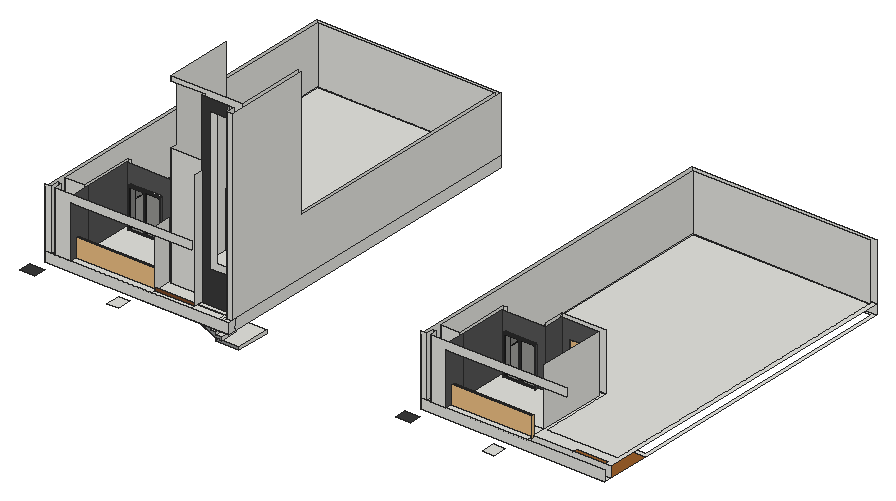
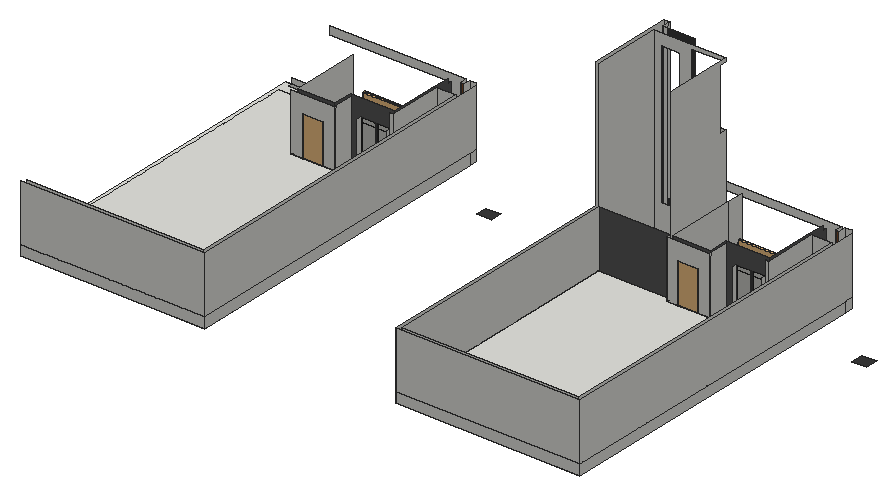
# SketchUp Ruby script. Lengths in inches.
U = 1.inch
M = Sketchup.active_model
def pt(a) = Geom::Point3d.new(a.map { |v| v * U })
def face(e, loops, mat)
  f = e.add_face(loops[0].map { |a| pt(a) })
  loops[1..].each { |l| e.add_face(l.map { |a| pt(a) }).erase! }
  f.material = f.back_material = mat if mat
  f
end
# faces: each face lists its corners as indices into pts; further lists are holes
def faces(e, pts, list, mat = nil) = list.each { |f| face(e, (f[0].is_a?(Array) ? f : [f]).map { |l| l.map { |i| pts[i] } }, mat) }
# xy, xz, yz: faces in a plane at the given z, y or x. An outline is a flat list of corners, or four numbers for a rectangle; further outlines are holes
def ring(l) = l.size == 4 ? [[l[0], l[1]], [l[2], l[1]], [l[2], l[3]], [l[0], l[3]]] : l.each_slice(2).to_a
def flat(e, list, mat, &to3) = list.each { |f| face(e, (f[0].is_a?(Array) ? f : [f]).map { |l| ring(l).map { |u, v| to3.(u, v) } }, mat) }
def xy(e, z, list, mat = nil) = flat(e, list, mat) { |x, y| [x, y, z] }
def xz(e, y, list, mat = nil) = flat(e, list, mat) { |x, z| [x, y, z] }
def yz(e, x, list, mat = nil) = flat(e, list, mat) { |y, z| [x, y, z] }
def lines(e, pts, list) = list.each { |a, b| e.add_line(pt(pts[a]), pt(pts[b])) }
# prism: a flat outline (further loops are holes) pulled along v
def prism(e, loops, v, mat = nil)
  f = face(e, loops, mat); d = Geom::Vector3d.new(v.map { |x| x * U })
  f.pushpull(f.normal.samedirection?(d) ? d.length : -d.length)
end
def box(e, o, s, mat = nil) = prism(e, [[o, [o[0] + s[0], o[1], o[2]], [o[0] + s[0], o[1] + s[1], o[2]], [o[0], o[1] + s[1], o[2]]]], [0, 0, s[2]], mat)
def at(x, y, z, deg = 0) = Geom::Transformation.translation(pt([x, y, z])) * Geom::Transformation.rotation(ORIGIN, Z_AXIS, deg.degrees)
def axes(o, x, y, z) = Geom::Transformation.new([*x, 0, *y, 0, *z, 0, *pt(o).to_a, 1])
def part(name) = M.definitions.add(name)
# library, detail: a bought-in or finely detailed component or shape, given as its bounding box
def library(name, o, s) = part(name).tap { |d| box(d.entities, o, s) }
def detail(e, o, s) = box(e.add_group.entities, o, s)
def put(e, d, t, mat = nil) = e.add_instance(d, t).tap { |i| i.material = mat if mat }
def group(e, t, mat = nil) = e.add_group.tap { |g| g.transformation = t; g.material = mat if mat }.entities
root = M.entities
M.materials.add("Glass_Tinted_Gray").color = [0, 0, 0]
M.materials["Glass_Tinted_Gray"].alpha = 0.125
M.materials.add("[0135_DarkGray]").color = [81, 81, 81]
M.materials.add("[Blacktop Old 02]").color = [143, 145, 145]
M.materials.add("[Color M06]").color = [86, 86, 86]
M.materials.add("[Color M07]").color = [58, 58, 58]
M.materials.add("[Mirror 02]").color = [229, 229, 229]
M.materials.add("[Terrazzo Light Blue]").color = [196, 214, 227]
M.materials.add("[Wood Floor Dark]").color = [153, 94, 42]
M.materials.add("[Wood Veneer 01]").color = [120, 70, 37]
c1 = part("PENTEK_RP Fineline 50S_Sliding_DoorCase_E1")
box(c1.entities,[0,0,0],[1.51,3.66,99.27],"[0135_DarkGray]")
c2 = part("PENTEK_RP Fineline 50S_SlidingDooe_Case_E2")
box(c2.entities,[0,0,0],[96.25,3.66,1.51],"[0135_DarkGray]")
c3 = part("pentek_RP Fineline 50S_SlidingDoor_Case")
put(c3.entities,c1,at(97.76,0,0))
put(c3.entities,c2,at(1.51,0,0))
put(c3.entities,c1,at(0,0,0))
put(c3.entities,c2,at(1.51,0,97.76))
c4 = part("PENTEK_RP Fineline 50S_SlidingDoor_GlazingBead_2")
box(c4.entities,[0,0,0],[0.56,0.59,94.39],"[0135_DarkGray]")
c5 = part("PENTEK_RP Fineline 50S_SlidingDoor_Glass")
box(c5.entities,[0,0,0],[46.58,0.16,94.39],"Glass_Tinted_Gray")
c6 = part("PENTEK_RP Fineline 50S_SlidingDoor_GlazingBead")
box(c6.entities,[0,0,0],[45.47,0.59,0.56],"[0135_DarkGray]")
c7 = part("PENTEK_RP Fineline 50S_SlidingDoor_Leaf_E1")
xy(c7.entities,0,[[0,0,0.93,1.97],[0.93,1.57,1.49,1.97]],"[0135_DarkGray]")
xy(c7.entities,96.25,[[0,0,0.93,0,0.93,1.57,1.49,1.57,1.49,1.97,0,1.97]],"[0135_DarkGray]")
xz(c7.entities,0,[[0,0,0.93,96.25]],"[0135_DarkGray]")
xz(c7.entities,1.57,[[0.93,0,1.49,95.32],[0.93,95.32,1.49,96.25]],"[0135_DarkGray]")
xz(c7.entities,1.97,[[0,0,1.49,96.25]],"[0135_DarkGray]")
yz(c7.entities,0,[[0,0,1.97,96.25]],"[0135_DarkGray]")
yz(c7.entities,0.93,[[0,0,1.57,0.93],[0,0.93,1.57,95.32],[0,95.32,1.57,96.25]],"[0135_DarkGray]")
yz(c7.entities,1.49,[[1.57,0,1.97,95.32],[1.57,95.32,1.97,96.25]],"[0135_DarkGray]")
c8 = part("PENTEK_RP Fineline 50S_SlidingDoor_Leaf_E2")
xy(c8.entities,0,[[0,0,0,1.57,0.56,1.57,0.56,1.97,46.02,1.97,46.02,1.57,46.58,1.57,46.58,0]],"[0135_DarkGray]")
xy(c8.entities,0.93,[[0,0,46.58,1.57]],"[0135_DarkGray]")
xy(c8.entities,1.49,[[0.56,1.57,46.02,1.97]],"[0135_DarkGray]")
xz(c8.entities,0,[[0,0,46.58,0.93]],"[0135_DarkGray]")
xz(c8.entities,1.57,[[0,0,0.56,0.93],[46.02,0,46.58,0.93],[0.56,0.93,46.02,1.49]],"[0135_DarkGray]")
xz(c8.entities,1.97,[[0.56,0,46.02,1.49]],"[0135_DarkGray]")
yz(c8.entities,0,[[0,0,1.57,0.93]],"[0135_DarkGray]")
yz(c8.entities,0.56,[[1.57,0,1.97,0.93],[1.57,0.93,1.97,1.49]],"[0135_DarkGray]")
yz(c8.entities,46.02,[[1.57,0,1.97,0.93],[1.57,0.93,1.97,1.49]],"[0135_DarkGray]")
yz(c8.entities,46.58,[[0,0,1.57,0.93]],"[0135_DarkGray]")
c9 = part("PENTEK_RP Fineline S_SlidingDoor_Leaf1")
put(c9.entities,c4,at(0.93,0,0.93))
put(c9.entities,c4,at(46.96,0,0.93))
put(c9.entities,c5,at(1.49,1.42,0.93))
put(c9.entities,c6,at(1.49,0,0.93))
put(c9.entities,c5,at(1.49,0.59,0.93),"[Terrazzo Light Blue]")
put(c9.entities,c7,at(0,0,0))
put(c9.entities,c7,axes([48.44,0,0],[-1,0,0],[0,1,0],[0,0,1]))
put(c9.entities,c8,axes([0.93,0,96.25],[1,0,0],[0,1,0],[0,0,-1]))
put(c9.entities,c8,at(0.93,0,0))
put(c9.entities,c6,at(1.49,0,94.77))
c10 = part("PENTEK_RP Fineline 50S_SlidingDoor_Leaf2")
put(c10.entities,c5,at(1.49,1.42,0.93))
put(c10.entities,c6,at(1.49,0,94.77))
put(c10.entities,c4,at(46.96,0,0.93))
put(c10.entities,c5,at(1.49,0.59,0.93),"[Mirror 02]")
put(c10.entities,c4,at(0.93,0,0.93))
put(c10.entities,c7,at(0,0,0))
put(c10.entities,c7,axes([48.44,0,0],[-1,0,0],[0,1,0],[0,0,1]))
put(c10.entities,c6,at(1.49,0,0.93))
put(c10.entities,c8,axes([0.93,0,96.25],[1,0,0],[0,1,0],[0,0,-1]))
put(c10.entities,c8,at(0.93,0,0))
c11 = part("PENTEK - Slimmest Steel Sliding Door / Window\#1")
put(c11.entities,c3,at(0,-1.88,-0.09))
put(c11.entities,c9,at(1.51,-2.27,1.42))
put(c11.entities,c10,at(49.32,-0.3,1.42))
c12 = library("Glass Railing",[0,0,0],[139.5,4.76,42])
c13 = library("door (1)",[38.93,25.48,0],[40,9.94,82.68])
xy(root,69.625,[[978.32,297.1875,1002.07,327.09],[1764.69,297.1875,1788.44,327.09]])
xy(root,69.625,[[796.71,297,827.45,321.97],[1583.09,297,1613.83,321.97]],"[Color M07]")
xy(root,71.875,[[1181.03,335.33,1193.03,371.33]])
xy(root,77.875,[[1205.03,299.33,1205.03,335.33,1217.03,335.33,1217.03,371.33,1253.03,371.33,1253.03,299.33],[1193.03,335.33,1205.03,371.33]])
xy(root,83.875,[[1205.03,299.33,1217.03,335.33],[1217.03,299.33,1253.03,299.33,1253.03,371.33,1205.03,371.33,1205.03,335.33,1217.03,335.33]])
xy(root,89.875,[[1205.03,299.33,1217.03,335.33]])
xy(root,94.0625,[[922.05,431.33,983.8,440.27],[1708.43,431.33,1770.18,440.27]])
xy(root,95.875,[[1193.03,299.33,1205.03,335.33]])
xy(root,101.875,[[1181.03,299.33,1193.03,335.33]])
xy(root,107.875,[[1169.03,299.33,1181.03,335.33]])
xy(root,113.875,[[1157.03,299.33,1169.03,335.33]])
xy(root,119.875,[[1145.03,299.33,1157.03,335.33]])
xy(root,125.875,[[874.71,264.125,1260.59,279.8125],[1661.09,264.125,2046.96,279.8125],[1133.03,299.33,1145.03,335.33],[[1061.03,371.33,1061.03,431.33,874.71,431.33,874.71,975.9375,1260.59,975.9375,1260.59,371.33],[1067.03,379.21,1255.32,379.21,1255.32,970.67,879.98,970.67,879.98,440.27,1067.03,440.27]],[[1847.4,371.33,1847.4,431.33,1661.09,431.33,1661.09,975.9375,2046.96,975.9375,2046.96,371.33],[1853.4,379.21,2041.7,379.21,2041.7,970.67,1666.35,970.67,1666.35,440.27,1853.4,440.27]]])
xy(root,125.875,[[[874.71,279.8125,874.71,431.33,1061.03,431.33,1061.03,371.33,1260.59,371.33,1260.59,279.8125],[1133.03,299.33,1145.03,335.33],[879.98,334.62,887.35,350.3]],[[1661.09,279.8125,1661.09,431.33,1847.4,431.33,1847.4,371.33,2046.96,371.33,2046.96,279.8125],[1919.4,299.33,1931.4,335.33],[1666.35,334.62,1673.73,350.3]]],"[Wood Floor Dark]")
xy(root,147.1875,[[881.96,308.24,881.96,968.69,1253.34,968.69,1253.34,452.5625,1103.7,452.5625,1103.7,462.67,1012.79,462.67,1012.79,420.39,971.61,421.04,922.07,421.04,922.07,308.24],[1668.33,308.24,1668.33,968.69,2039.72,968.69,2039.72,452.5625,1890.08,452.5625,1890.08,462.67,1799.16,462.67,1799.16,420.39,1757.99,421.04,1708.45,421.04,1708.45,308.24]])
xy(root,147.625,[[874.71,264.125,888.27,279.8125],[888.27,264.125,895.625,279.8125],[895.625,264.125,928.09,279.8125],[928.09,264.125,1098.03,279.8125],[1098.03,264.125,1181.97,272.125],
  [1181.97,264.125,1239.03,279.8125],[1239.03,264.125,1245.07,279.8125],[1245.07,264.125,1249.29,264.125,1249.29,273.0625,1245.07,279.8125],[1249.29,264.125,1260.59,273.0625],[1661.09,264.125,1674.65,279.8125],
  [1674.65,264.125,1682,279.8125],[1682,264.125,1714.47,279.8125],[1714.47,264.125,1884.4,279.8125],[1098.03,272.125,1181.97,273.0625],[1098.03,273.0625,1181.97,279.8125],
  [1249.29,273.0625,1249.29,279.8125,1245.07,279.8125],[1249.29,273.0625,1260.59,279.8125],[874.71,279.8125,874.71,975.9375,1260.59,975.9375,1260.59,279.8125,1249.29,279.8125,1249.29,289.5,1181.97,289.5,1181.97,279.8125,1098.03,279.8125,1098.03,452.5625,1079.72,452.5625,1079.72,462.67,1103.7,462.67,1103.7,308.24,1253.34,308.24,1253.34,968.69,881.96,968.69,881.96,308.24,922.07,308.24,922.07,421.04,937.22,421.04,937.22,411.0625,928.09,411.0625,928.09,279.8125],[928.09,279.8125,1098.03,308.24],[1181.97,279.8125,1239.03,289.5],
  [1239.03,279.8125,1245.07,279.8125,1239.03,289.5],[1245.07,279.8125,1239.03,289.5,1249.29,289.5,1249.29,279.8125],[1661.09,279.8125,1661.09,975.9375,2046.96,975.9375,2046.96,279.8125,2035.66,279.8125,2035.66,289.5,1968.34,289.5,1968.34,279.8125,1884.4,279.8125,1884.4,452.5625,1866.1,452.5625,1866.1,462.67,1890.08,462.67,1890.08,308.24,2039.72,308.24,2039.72,968.69,1668.33,968.69,1668.33,308.24,1708.45,308.24,1708.45,421.04,1723.6,421.04,1723.6,411.0625,1714.47,411.0625,1714.47,279.8125],[1714.47,279.8125,1884.4,308.24],[881.96,308.24,881.96,968.69,1253.34,968.69,1253.34,308.24,1103.7,308.24,1103.7,462.67,1012.79,462.67,1012.79,420.39,998.97,420.61,971.61,421.04,922.07,421.04,922.07,308.24],
  [928.09,308.24,1098.03,308.24,1098.03,452.5625,1079.72,452.5625,1079.72,462.67,1037.97,462.67,1037.97,452.5625,1019.84,452.5625,1019.84,411.0625,998.97,411.0625,998.97,420.61,937.22,420.61,937.22,411.0625,928.09,411.0625],[1668.33,308.24,1668.33,968.69,2039.72,968.69,2039.72,308.24,1890.08,308.24,1890.08,462.67,1799.16,462.67,1799.16,420.39,1785.35,420.61,1757.99,421.04,1708.45,421.04,1708.45,308.24],[1714.47,308.24,1884.4,308.24,1884.4,452.5625,1866.1,452.5625,1866.1,462.67,1824.35,462.67,1824.35,452.5625,1806.22,452.5625,1806.22,411.0625,1785.35,411.0625,1785.35,420.61,1723.6,420.61,1723.6,411.0625,1714.47,411.0625],[998.97,411.0625,998.97,420.61,1012.79,420.39,1012.79,462.67,1037.97,462.67,1037.97,452.5625,1019.84,452.5625,1019.84,411.0625],[1785.35,411.0625,1785.35,420.61,1799.16,420.39,1799.16,462.67,1824.35,462.67,1824.35,452.5625,1806.22,452.5625,1806.22,411.0625],
  [937.22,420.61,937.22,421.04,971.61,421.04,998.97,420.61],[1723.6,420.61,1723.6,421.04,1757.99,421.04,1785.35,420.61]])
xz(root,264.125,[[874.71,125.875,1260.59,147.625],[1661.09,125.875,2046.96,147.625],[874.71,147.625,888.27,273.625],[895.625,147.625,928.09,147.625,928.09,256.875,1181.97,256.875,1181.97,273.625,895.625,273.625],[1661.09,147.625,1674.65,273.625],
  [1682,147.625,1714.47,147.625,1714.47,256.875,1968.34,256.875,1968.34,273.625,1682,273.625]])
xz(root,272.125,[[1098.03,147.625,1181.97,154.375]],"[Wood Veneer 01]")
xz(root,273.0625,[[1098.03,143.05,1181.97,147.625],[1249.29,147.625,1260.59,536.4375]])
xz(root,279.8125,[[874.71,125.875,1260.59,147.625],[1661.09,125.875,2046.96,147.625]])
xz(root,279.8125,[[888.27,147.625,895.625,273.625],[1674.65,147.625,1682,273.625]],"[Wood Veneer 01]")
xz(root,289.5,[[1239.03,147.625,1249.29,536.4375]])
xz(root,289.5,[[1181.97,147.625,1239.03,147.625,1239.03,217.36,1200.15,217.36,1200.15,512.23,1239.03,512.23,1239.03,536.4375,1181.97,536.4375]],"[Color M07]")
xz(root,299.33,[[1205.03,77.875,1253.03,83.875],[1205.03,83.875,1217.03,83.875,1217.03,89.875,1205.03,89.875,1205.03,95.875,1193.03,95.875,1193.03,101.875,1181.03,101.875,1181.03,107.875,1169.03,107.875,1169.03,113.875,1157.03,113.875,1157.03,119.875,1145.03,119.875,1145.03,125.875,1133.03,125.875,1133.03,119.875]],"[Blacktop Old 02]")
xz(root,308.24,[[881.96,147.1875,922.07,147.625],[1668.33,147.1875,1708.45,147.625],[881.96,147.625,922.07,267.625],[[1103.7,147.625,1103.7,400.68,1175.84,400.68,1175.84,528.11,1103.7,528.11,1103.7,536.4375,1253.34,536.4375,1253.34,147.625],[1200.15,217.36,1239.03,512.23]],[1668.33,147.625,1708.45,267.625]])
xz(root,335.33,[[1205.03,83.875,1133.03,119.875,1133.03,125.875,1145.03,125.875,1145.03,119.875,1157.03,119.875,1157.03,113.875,1169.03,113.875,1169.03,107.875,1181.03,107.875,1181.03,101.875,1193.03,101.875,1193.03,95.875,1205.03,95.875,1205.03,89.875,1217.03,89.875,1217.03,83.875]])
xz(root,411.0625,[[928.09,147.625,937.22,147.625,937.22,230.5625,998.97,230.5625,998.97,147.625,1019.84,147.625,1019.84,267.625,928.09,267.625],[1714.47,147.625,1723.6,147.625,1723.6,230.5625,1785.35,230.5625,1785.35,147.625,1806.22,147.625,1806.22,267.625,1714.47,267.625]],"[Color M06]")
xz(root,421.04,[[922.07,147.1875,929.34,147.625],[929.34,147.1875,971.61,147.625],[1708.45,147.1875,1715.71,147.625],[1715.71,147.1875,1757.99,147.625],[922.07,147.625,929.34,267.625],
  [1708.45,147.625,1715.71,267.625]])
xz(root,452.5625,[[1103.7,147.1875,1253.34,267.625],[1019.84,147.625,1037.97,147.625,1037.97,231.75,1079.72,231.75,1079.72,147.625,1098.03,147.625,1098.03,267.625,1019.84,267.625],[1806.22,147.625,1824.35,147.625,1824.35,231.75,1866.1,231.75,1866.1,147.625,1884.4,147.625,1884.4,267.625,1806.22,267.625]],"[Color M06]")
xz(root,462.67,[[1012.79,147.1875,1103.7,147.625],[1799.16,147.1875,1890.08,147.625],[1012.79,147.625,1037.97,147.625,1037.97,231.75,1079.72,231.75,1079.72,147.625,1103.7,147.625,1103.7,267.625,1012.79,267.625],[1799.16,147.625,1824.35,147.625,1824.35,231.75,1866.1,231.75,1866.1,147.625,1890.08,147.625,1890.08,267.625,1799.16,267.625]])
xz(root,968.69,[[881.96,147.1875,1253.34,147.625],[1668.33,147.1875,2039.72,147.625],[881.96,147.625,1253.34,267.625],[1668.33,147.625,2039.72,267.625]])
xz(root,975.9375,[[874.71,125.875,1260.59,147.625],[1661.09,125.875,2046.96,147.625],[874.71,147.625,1260.59,267.625],[1661.09,147.625,2046.96,267.625]])
yz(root,874.71,[[264.125,125.875,279.8125,147.625],[279.8125,125.875,975.9375,147.625],[264.125,147.625,975.9375,267.625]])
yz(root,881.96,[[308.24,147.1875,968.69,147.625],[308.24,147.625,968.69,267.625]])
yz(root,888.27,[[264.125,147.625,279.8125,273.625]])
yz(root,895.625,[[264.125,147.625,279.8125,273.625]])
yz(root,922.07,[[308.24,147.1875,421.04,147.625],[308.24,147.625,421.04,267.625]])
yz(root,928.09,[[264.125,147.625,308.24,147.625,308.24,267.625,272.68,267.625,272.68,256.875,264.125,256.875],[308.24,147.625,411.0625,267.625]],"[Color M06]")
yz(root,937.22,[[411.0625,147.625,420.61,230.5625]])
yz(root,998.97,[[411.0625,147.625,420.61,230.5625]])
yz(root,1012.79,[[420.39,147.1875,459.32,147.625],[459.32,147.1875,462.67,147.625],[420.39,147.625,459.32,267.625],[459.32,147.625,462.67,267.625]])
yz(root,1019.84,[[411.0625,147.625,452.5625,267.625]],"[Color M06]")
yz(root,1037.97,[[452.5625,147.625,462.67,231.75]])
yz(root,1079.72,[[452.5625,147.625,462.67,231.75]])
yz(root,1098.03,[[272.125,147.625,272.125,154.375,273.0625,154.375,273.0625,155.86,272.125,155.86,272.125,167.1875,273.0625,167.1875,273.0625,168.67,272.125,168.67,272.125,180,273.0625,180,273.0625,181.48,272.125,181.48,272.125,192.8125,273.0625,192.8125,273.0625,194.3,272.125,194.3,272.125,205.625,273.0625,205.625,273.0625,207.11,272.125,207.11,272.125,218.4375,273.0625,218.4375,273.0625,219.92,272.125,219.92,272.125,231.25,273.0625,231.25,273.0625,232.73,272.125,232.73,272.125,244.0625,273.0625,244.0625,273.0625,245.55,272.125,245.55,272.125,256.875,273.0625,256.875,273.0625,267.625,308.24,267.625,308.24,147.625],[308.24,147.625,452.5625,267.625]])
yz(root,1103.7,[[452.5625,147.1875,462.67,147.625],[308.24,147.625,452.5625,147.625,452.5625,536.4375,308.24,536.4375,308.24,528.11,323.81,528.11,323.81,400.68,308.24,400.68],[452.5625,147.625,462.67,267.625]])
yz(root,1133.03,[[299.33,119.875,335.33,125.875]])
yz(root,1145.03,[[299.33,119.875,335.33,125.875]])
yz(root,1157.03,[[299.33,113.875,335.33,119.875]])
yz(root,1169.03,[[299.33,107.875,335.33,113.875]])
yz(root,1181.03,[[299.33,101.875,335.33,107.875]])
yz(root,1181.97,[[272.125,147.625,289.5,147.625,289.5,393.625,271.6875,393.625,271.6875,273.625,273.0625,273.625,273.0625,256.875,272.125,256.875,272.125,245.55,273.0625,245.55,273.0625,244.0625,272.125,244.0625,272.125,232.73,273.0625,232.73,273.0625,231.25,272.125,231.25,272.125,219.92,273.0625,219.92,273.0625,218.4375,272.125,218.4375,272.125,207.11,273.0625,207.11,273.0625,205.625,272.125,205.625,272.125,194.3,273.0625,194.3,273.0625,192.8125,272.125,192.8125,272.125,181.48,273.0625,181.48,273.0625,180,272.125,180,272.125,168.67,273.0625,168.67,273.0625,167.1875,272.125,167.1875,272.125,155.86,273.0625,155.86,273.0625,154.375,272.125,154.375]])
yz(root,1193.03,[[299.33,95.875,335.33,101.875]])
yz(root,1193.03,[[335.33,71.875,371.33,77.875]],"[Blacktop Old 02]")
yz(root,1205.03,[[299.33,89.875,335.33,95.875]])
yz(root,1205.03,[[299.33,77.875,335.33,83.875],[335.33,77.875,371.33,83.875]],"[Blacktop Old 02]")
yz(root,1217.03,[[299.33,83.875,335.33,89.875]])
yz(root,1249.29,[[273.0625,147.625,289.5,536.4375]])
yz(root,1253.03,[[299.33,77.875,371.33,83.875]])
yz(root,1253.34,[[452.5625,147.1875,968.69,147.625],[308.24,147.625,452.5625,536.4375],[452.5625,147.625,968.69,267.625]])
yz(root,1260.59,[[264.125,125.875,279.8125,147.625],[279.8125,125.875,975.9375,147.625],[273.0625,147.625,975.9375,147.625,975.9375,267.625,452.5625,267.625,452.5625,536.4375,273.0625,536.4375]])
yz(root,1661.09,[[264.125,125.875,279.8125,147.625],[279.8125,125.875,975.9375,147.625],[264.125,147.625,975.9375,267.625]])
yz(root,1668.33,[[308.24,147.1875,968.69,147.625],[308.24,147.625,968.69,267.625]])
yz(root,1674.65,[[264.125,147.625,279.8125,273.625]])
yz(root,1682,[[264.125,147.625,279.8125,273.625]])
yz(root,1708.45,[[308.24,147.1875,421.04,147.625],[308.24,147.625,421.04,267.625]])
yz(root,1714.47,[[264.125,147.625,308.24,147.625,308.24,267.625,272.68,267.625,272.68,256.875,264.125,256.875],[308.24,147.625,411.0625,267.625]],"[Color M06]")
yz(root,1723.6,[[411.0625,147.625,420.61,230.5625]])
yz(root,1785.35,[[411.0625,147.625,420.61,230.5625]])
yz(root,1799.16,[[420.39,147.1875,459.32,147.625],[459.32,147.1875,462.67,147.625],[420.39,147.625,459.32,267.625],[459.32,147.625,462.67,267.625]])
yz(root,1806.22,[[411.0625,147.625,452.5625,267.625]],"[Color M06]")
yz(root,1824.35,[[452.5625,147.625,462.67,231.75]])
yz(root,1866.1,[[452.5625,147.625,462.67,231.75]])
yz(root,1884.4,[[308.24,147.625,452.5625,267.625]])
p = [[1133.03,335.33,119.875],[1205.03,335.33,83.875],[1205.03,299.33,83.875],[1133.03,299.33,119.875],[1012.79,420.39,147.1875],[1012.79,420.39,147.625],
  [998.97,420.61,147.625],[971.61,421.04,147.625],[971.61,421.04,147.1875],[1799.16,420.39,147.1875],[1799.16,420.39,147.625],[1785.35,420.61,147.625],
  [1757.99,421.04,147.625],[1757.99,421.04,147.1875],[1249.29,273.0625,536.4375],[1239.03,289.5,536.4375],[1239.03,289.5,512.23],[1239.03,289.5,217.36],
  [1239.03,289.5,147.625],[1245.07,279.8125,147.625],[1249.29,273.0625,147.625],[1133.03,335.33,131.875],[1121.03,335.33,131.875],[1133.03,335.33,125.875]]
faces(root,p,[[0,1,2,3]],"[Blacktop Old 02]")
faces(root,p,[[4,5,6,7,8],[9,10,11,12,13],[14,15,16,17,18,19,20]])
lines(root,p,[[21,22],[23,21]])
put(root,c11,axes([936.27,405.56,146.3],[0.6868,0,0],[0,0.6868,0],[0,0,0.85163]))
put(root,c12,axes([927.52,277.75,143.83],[1.22225,0,0],[0,1,0],[0,0,1]))
put(root,c13,axes([997.34,427.08,147.625],[1.04375,0,0],[0,1,0],[0,0,1.01751]))
put(root,c11,axes([1722.64,405.56,146.3],[0.6868,0,0],[0,0.6868,0],[0,0,0.85163]))
put(root,c12,axes([1713.9,277.75,143.83],[1.22225,0,0],[0,1,0],[0,0,1]))
put(root,c13,axes([1783.71,427.08,147.625],[1.04375,0,0],[0,1,0],[0,0,1.01751]))
